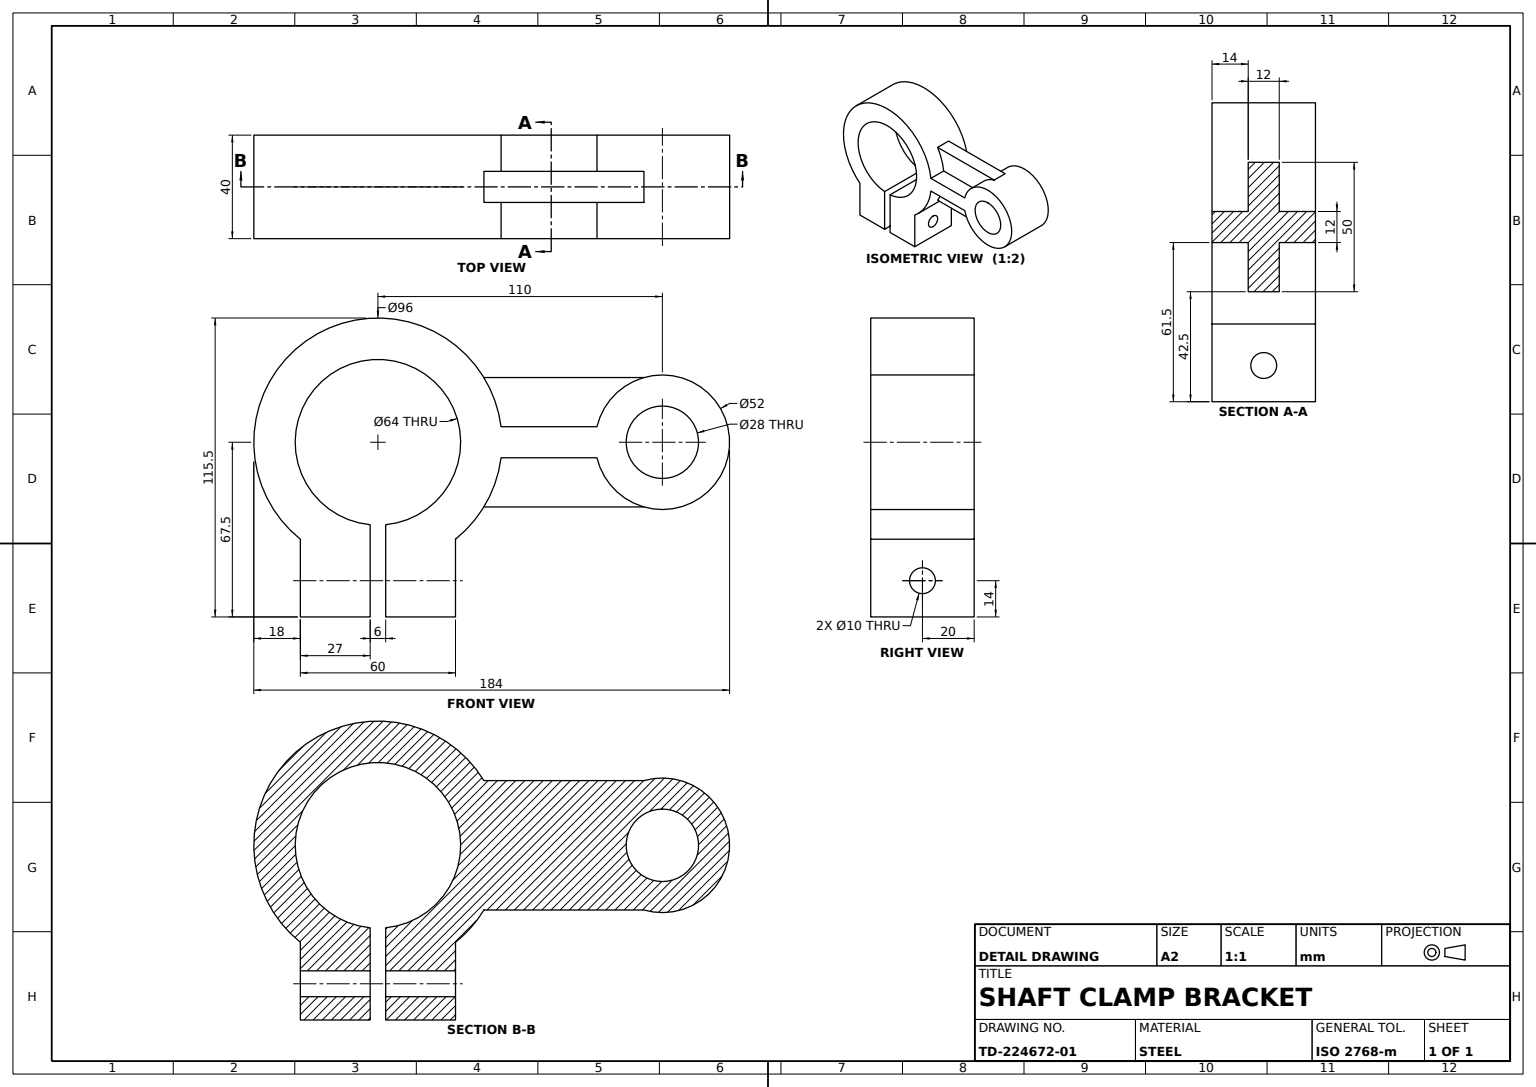
ISO-10303-21;
HEADER;
FILE_DESCRIPTION((''),'2;1');
FILE_NAME('','',(''),(''),'','','');
FILE_SCHEMA(('AUTOMOTIVE_DESIGN'));
ENDSEC;
DATA;
#1=APPLICATION_CONTEXT('');
#2=PRODUCT_CONTEXT('',#1,'mechanical');
#3=PRODUCT('','','',(#2));
#4=PRODUCT_DEFINITION_FORMATION('','',#3);
#5=PRODUCT_DEFINITION_CONTEXT('',#1,'design');
#6=PRODUCT_DEFINITION('','',#4,#5);
#7=PRODUCT_DEFINITION_SHAPE('','',#6);
#8=(LENGTH_UNIT()NAMED_UNIT(*)SI_UNIT(.MILLI.,.METRE.));
#9=(NAMED_UNIT(*)PLANE_ANGLE_UNIT()SI_UNIT($,.RADIAN.));
#10=(NAMED_UNIT(*)SI_UNIT($,.STERADIAN.)SOLID_ANGLE_UNIT());
#11=UNCERTAINTY_MEASURE_WITH_UNIT(LENGTH_MEASURE(0.005),#8,'distance_accuracy_value','');
#12=(GEOMETRIC_REPRESENTATION_CONTEXT(3)GLOBAL_UNCERTAINTY_ASSIGNED_CONTEXT((#11))GLOBAL_UNIT_ASSIGNED_CONTEXT((#8,#9,#10))REPRESENTATION_CONTEXT('',''));
#13=CARTESIAN_POINT('',(40.975602,-6.,-25.));
#14=VERTEX_POINT('',#13);
#15=CARTESIAN_POINT('',(40.975602,6.,-25.));
#16=VERTEX_POINT('',#15);
#17=CARTESIAN_POINT('',(40.975602,-20.,-25.));
#18=DIRECTION('',(0.,1.,0.));
#19=VECTOR('',#18,1000.);
#20=LINE('',#17,#19);
#21=EDGE_CURVE('',#14,#16,#20,.T.);
#22=ORIENTED_EDGE('',*,*,#21,.T.);
#23=CARTESIAN_POINT('',(102.858572,6.,-25.));
#24=VERTEX_POINT('',#23);
#25=CARTESIAN_POINT('',(35.,6.,-25.));
#26=DIRECTION('',(1.,0.,0.));
#27=VECTOR('',#26,1000.);
#28=LINE('',#25,#27);
#29=EDGE_CURVE('',#16,#24,#28,.T.);
#30=ORIENTED_EDGE('',*,*,#29,.T.);
#31=CARTESIAN_POINT('',(102.858572,-6.,-25.));
#32=VERTEX_POINT('',#31);
#33=CARTESIAN_POINT('',(102.858572,-20.,-25.));
#34=LINE('',#33,#19);
#35=EDGE_CURVE('',#32,#24,#34,.T.);
#36=ORIENTED_EDGE('',*,*,#35,.F.);
#37=CARTESIAN_POINT('',(35.,-6.,-25.));
#38=LINE('',#37,#27);
#39=EDGE_CURVE('',#14,#32,#38,.T.);
#40=ORIENTED_EDGE('',*,*,#39,.F.);
#41=EDGE_LOOP('',(#22,#30,#36,#40));
#42=FACE_BOUND('',#41,.T.);
#43=DIRECTION('',(0.,0.,1.));
#44=AXIS2_PLACEMENT_3D('',#37,#43,#26);
#45=PLANE('',#44);
#46=ADVANCED_FACE('',(#42),#45,.F.);
#47=CARTESIAN_POINT('',(30.,-20.,-37.469988));
#48=VERTEX_POINT('',#47);
#49=CARTESIAN_POINT('',(30.,20.,-37.469988));
#50=VERTEX_POINT('',#49);
#51=LINE('',#47,#19);
#52=EDGE_CURVE('',#48,#50,#51,.T.);
#53=ORIENTED_EDGE('',*,*,#52,.F.);
#54=CARTESIAN_POINT('',(30.,-20.,-67.5));
#55=VERTEX_POINT('',#54);
#56=VECTOR('',#43,1000.);
#57=LINE('',#54,#56);
#58=EDGE_CURVE('',#55,#48,#57,.T.);
#59=ORIENTED_EDGE('',*,*,#58,.F.);
#60=CARTESIAN_POINT('',(30.,20.,-67.5));
#61=VERTEX_POINT('',#60);
#62=LINE('',#54,#19);
#63=EDGE_CURVE('',#55,#61,#62,.T.);
#64=ORIENTED_EDGE('',*,*,#63,.T.);
#65=LINE('',#60,#56);
#66=EDGE_CURVE('',#61,#50,#65,.T.);
#67=ORIENTED_EDGE('',*,*,#66,.T.);
#68=EDGE_LOOP('',(#53,#59,#64,#67));
#69=FACE_BOUND('',#68,.T.);
#70=CARTESIAN_POINT('',(30.,0.,-48.5));
#71=VERTEX_POINT('',#70);
#72=CARTESIAN_POINT('',(30.,0.,-53.5));
#73=DIRECTION('',(-1.,0.,0.));
#74=AXIS2_PLACEMENT_3D('',#72,#73,#43);
#75=CIRCLE('',#74,5.);
#76=EDGE_CURVE('',#71,#71,#75,.T.);
#77=ORIENTED_EDGE('',*,*,#76,.T.);
#78=EDGE_LOOP('',(#77));
#79=FACE_BOUND('',#78,.T.);
#80=AXIS2_PLACEMENT_3D('',#54,#73,#43);
#81=PLANE('',#80);
#82=ADVANCED_FACE('',(#69,#79),#81,.F.);
#83=CARTESIAN_POINT('',(-30.,20.,-67.5));
#84=VERTEX_POINT('',#83);
#85=CARTESIAN_POINT('',(-3.,20.,-67.5));
#86=VERTEX_POINT('',#85);
#87=LINE('',#83,#27);
#88=EDGE_CURVE('',#84,#86,#87,.T.);
#89=ORIENTED_EDGE('',*,*,#88,.T.);
#90=CARTESIAN_POINT('',(-3.,-20.,-67.5));
#91=VERTEX_POINT('',#90);
#92=DIRECTION('',(0.,-1.,0.));
#93=VECTOR('',#92,1000.);
#94=LINE('',#90,#93);
#95=EDGE_CURVE('',#86,#91,#94,.T.);
#96=ORIENTED_EDGE('',*,*,#95,.T.);
#97=CARTESIAN_POINT('',(-30.,-20.,-67.5));
#98=VERTEX_POINT('',#97);
#99=LINE('',#97,#27);
#100=EDGE_CURVE('',#98,#91,#99,.T.);
#101=ORIENTED_EDGE('',*,*,#100,.F.);
#102=LINE('',#97,#19);
#103=EDGE_CURVE('',#98,#84,#102,.T.);
#104=ORIENTED_EDGE('',*,*,#103,.T.);
#105=EDGE_LOOP('',(#89,#96,#101,#104));
#106=FACE_BOUND('',#105,.T.);
#107=AXIS2_PLACEMENT_3D('',#97,#43,#26);
#108=PLANE('',#107);
#109=ADVANCED_FACE('',(#106),#108,.F.);
#110=CARTESIAN_POINT('',(-3.,0.,-48.5));
#111=VERTEX_POINT('',#110);
#112=CARTESIAN_POINT('',(-3.,0.,-53.5));
#113=AXIS2_PLACEMENT_3D('',#112,#73,#43);
#114=CIRCLE('',#113,5.);
#115=EDGE_CURVE('',#111,#111,#114,.T.);
#116=ORIENTED_EDGE('',*,*,#115,.F.);
#117=EDGE_LOOP('',(#116));
#118=FACE_BOUND('',#117,.T.);
#119=CARTESIAN_POINT('',(-30.,0.,-58.5));
#120=VERTEX_POINT('',#119);
#121=CARTESIAN_POINT('',(-30.,0.,-53.5));
#122=DIRECTION('',(0.,0.,-1.));
#123=AXIS2_PLACEMENT_3D('',#121,#26,#122);
#124=CIRCLE('',#123,5.);
#125=EDGE_CURVE('',#120,#120,#124,.T.);
#126=ORIENTED_EDGE('',*,*,#125,.F.);
#127=EDGE_LOOP('',(#126));
#128=FACE_BOUND('',#127,.T.);
#129=CYLINDRICAL_SURFACE('',#74,5.);
#130=ADVANCED_FACE('',(#118,#128),#129,.F.);
#131=CARTESIAN_POINT('',(-3.,20.,-31.859065));
#132=VERTEX_POINT('',#131);
#133=CARTESIAN_POINT('',(-3.,-20.,-31.859065));
#134=VERTEX_POINT('',#133);
#135=LINE('',#133,#19);
#136=EDGE_CURVE('',#132,#134,#135,.F.);
#137=ORIENTED_EDGE('',*,*,#136,.F.);
#138=CARTESIAN_POINT('',(3.,20.,-31.859065));
#139=VERTEX_POINT('',#138);
#140=CARTESIAN_POINT('',(0.,20.,0.));
#141=AXIS2_PLACEMENT_3D('',#140,#92,#122);
#142=CIRCLE('',#141,32.);
#143=EDGE_CURVE('',#139,#132,#142,.T.);
#144=ORIENTED_EDGE('',*,*,#143,.F.);
#145=CARTESIAN_POINT('',(3.,-20.,-31.859065));
#146=VERTEX_POINT('',#145);
#147=LINE('',#145,#19);
#148=EDGE_CURVE('',#146,#139,#147,.T.);
#149=ORIENTED_EDGE('',*,*,#148,.F.);
#150=CARTESIAN_POINT('',(0.,-20.,0.));
#151=AXIS2_PLACEMENT_3D('',#150,#18,#43);
#152=CIRCLE('',#151,32.);
#153=EDGE_CURVE('',#134,#146,#152,.T.);
#154=ORIENTED_EDGE('',*,*,#153,.F.);
#155=EDGE_LOOP('',(#137,#144,#149,#154));
#156=FACE_BOUND('',#155,.T.);
#157=CYLINDRICAL_SURFACE('',#151,32.);
#158=ADVANCED_FACE('',(#156),#157,.F.);
#159=CARTESIAN_POINT('',(84.701779,6.,-6.));
#160=VERTEX_POINT('',#159);
#161=CARTESIAN_POINT('',(47.623524,6.,-6.));
#162=VERTEX_POINT('',#161);
#163=CARTESIAN_POINT('',(0.,6.,-6.));
#164=VECTOR('',#73,1000.);
#165=LINE('',#163,#164);
#166=EDGE_CURVE('',#160,#162,#165,.T.);
#167=ORIENTED_EDGE('',*,*,#166,.T.);
#168=CARTESIAN_POINT('',(47.623524,20.,-6.));
#169=VERTEX_POINT('',#168);
#170=CARTESIAN_POINT('',(47.623524,-20.,-6.));
#171=LINE('',#170,#19);
#172=EDGE_CURVE('',#162,#169,#171,.T.);
#173=ORIENTED_EDGE('',*,*,#172,.T.);
#174=CARTESIAN_POINT('',(84.701779,20.,-6.));
#175=VERTEX_POINT('',#174);
#176=CARTESIAN_POINT('',(90.,20.,-6.));
#177=LINE('',#176,#164);
#178=EDGE_CURVE('',#175,#169,#177,.T.);
#179=ORIENTED_EDGE('',*,*,#178,.F.);
#180=CARTESIAN_POINT('',(84.701779,-20.,-6.));
#181=LINE('',#180,#19);
#182=EDGE_CURVE('',#175,#160,#181,.F.);
#183=ORIENTED_EDGE('',*,*,#182,.T.);
#184=EDGE_LOOP('',(#167,#173,#179,#183));
#185=FACE_BOUND('',#184,.T.);
#186=CARTESIAN_POINT('',(0.,0.,-6.));
#187=AXIS2_PLACEMENT_3D('',#186,#43,#26);
#188=PLANE('',#187);
#189=ADVANCED_FACE('',(#185),#188,.F.);
#190=CARTESIAN_POINT('',(40.975602,6.,25.));
#191=VERTEX_POINT('',#190);
#192=CARTESIAN_POINT('',(40.975602,-6.,25.));
#193=VERTEX_POINT('',#192);
#194=CARTESIAN_POINT('',(40.975602,-20.,25.));
#195=LINE('',#194,#19);
#196=EDGE_CURVE('',#191,#193,#195,.F.);
#197=ORIENTED_EDGE('',*,*,#196,.T.);
#198=CARTESIAN_POINT('',(102.858572,-6.,25.));
#199=VERTEX_POINT('',#198);
#200=CARTESIAN_POINT('',(110.,-6.,25.));
#201=LINE('',#200,#164);
#202=EDGE_CURVE('',#199,#193,#201,.T.);
#203=ORIENTED_EDGE('',*,*,#202,.F.);
#204=CARTESIAN_POINT('',(102.858572,6.,25.));
#205=VERTEX_POINT('',#204);
#206=CARTESIAN_POINT('',(102.858572,-20.,25.));
#207=LINE('',#206,#19);
#208=EDGE_CURVE('',#205,#199,#207,.F.);
#209=ORIENTED_EDGE('',*,*,#208,.F.);
#210=CARTESIAN_POINT('',(110.,6.,25.));
#211=LINE('',#210,#164);
#212=EDGE_CURVE('',#205,#191,#211,.T.);
#213=ORIENTED_EDGE('',*,*,#212,.T.);
#214=EDGE_LOOP('',(#197,#203,#209,#213));
#215=FACE_BOUND('',#214,.T.);
#216=AXIS2_PLACEMENT_3D('',#200,#122,#73);
#217=PLANE('',#216);
#218=ADVANCED_FACE('',(#215),#217,.F.);
#219=CARTESIAN_POINT('',(110.,-20.,14.));
#220=VERTEX_POINT('',#219);
#221=CARTESIAN_POINT('',(110.,-20.,0.));
#222=AXIS2_PLACEMENT_3D('',#221,#18,#43);
#223=CIRCLE('',#222,14.);
#224=EDGE_CURVE('',#220,#220,#223,.T.);
#225=ORIENTED_EDGE('',*,*,#224,.F.);
#226=EDGE_LOOP('',(#225));
#227=FACE_BOUND('',#226,.T.);
#228=CARTESIAN_POINT('',(110.,20.,-14.));
#229=VERTEX_POINT('',#228);
#230=CARTESIAN_POINT('',(110.,20.,0.));
#231=AXIS2_PLACEMENT_3D('',#230,#92,#122);
#232=CIRCLE('',#231,14.);
#233=EDGE_CURVE('',#229,#229,#232,.T.);
#234=ORIENTED_EDGE('',*,*,#233,.F.);
#235=EDGE_LOOP('',(#234));
#236=FACE_BOUND('',#235,.T.);
#237=CYLINDRICAL_SURFACE('',#222,14.);
#238=ADVANCED_FACE('',(#227,#236),#237,.F.);
#239=CARTESIAN_POINT('',(3.,-20.,-67.5));
#240=VERTEX_POINT('',#239);
#241=CARTESIAN_POINT('',(3.,20.,-67.5));
#242=VERTEX_POINT('',#241);
#243=LINE('',#239,#19);
#244=EDGE_CURVE('',#240,#242,#243,.T.);
#245=ORIENTED_EDGE('',*,*,#244,.F.);
#246=CARTESIAN_POINT('',(3.,-20.,0.));
#247=LINE('',#246,#56);
#248=EDGE_CURVE('',#240,#146,#247,.T.);
#249=ORIENTED_EDGE('',*,*,#248,.T.);
#250=ORIENTED_EDGE('',*,*,#148,.T.);
#251=CARTESIAN_POINT('',(3.,20.,0.));
#252=LINE('',#251,#56);
#253=EDGE_CURVE('',#242,#139,#252,.T.);
#254=ORIENTED_EDGE('',*,*,#253,.F.);
#255=EDGE_LOOP('',(#245,#249,#250,#254));
#256=FACE_BOUND('',#255,.T.);
#257=CARTESIAN_POINT('',(3.,0.,-58.5));
#258=VERTEX_POINT('',#257);
#259=CARTESIAN_POINT('',(3.,0.,-53.5));
#260=AXIS2_PLACEMENT_3D('',#259,#26,#122);
#261=CIRCLE('',#260,5.);
#262=EDGE_CURVE('',#258,#258,#261,.T.);
#263=ORIENTED_EDGE('',*,*,#262,.T.);
#264=EDGE_LOOP('',(#263));
#265=FACE_BOUND('',#264,.T.);
#266=CARTESIAN_POINT('',(3.,-25.,-30.384328));
#267=AXIS2_PLACEMENT_3D('',#266,#26,#122);
#268=PLANE('',#267);
#269=ADVANCED_FACE('',(#256,#265),#268,.F.);
#270=ORIENTED_EDGE('',*,*,#208,.T.);
#271=CARTESIAN_POINT('',(84.701779,-6.,6.));
#272=VERTEX_POINT('',#271);
#273=CARTESIAN_POINT('',(110.,-6.,0.));
#274=AXIS2_PLACEMENT_3D('',#273,#92,#122);
#275=CIRCLE('',#274,26.);
#276=EDGE_CURVE('',#272,#199,#275,.F.);
#277=ORIENTED_EDGE('',*,*,#276,.F.);
#278=CARTESIAN_POINT('',(84.701779,-20.,6.));
#279=VERTEX_POINT('',#278);
#280=LINE('',#278,#19);
#281=EDGE_CURVE('',#272,#279,#280,.F.);
#282=ORIENTED_EDGE('',*,*,#281,.T.);
#283=VERTEX_POINT('',#180);
#284=AXIS2_PLACEMENT_3D('',#221,#92,#26);
#285=CIRCLE('',#284,26.);
#286=EDGE_CURVE('',#283,#279,#285,.T.);
#287=ORIENTED_EDGE('',*,*,#286,.F.);
#288=CARTESIAN_POINT('',(84.701779,-6.,-6.));
#289=VERTEX_POINT('',#288);
#290=EDGE_CURVE('',#289,#283,#181,.F.);
#291=ORIENTED_EDGE('',*,*,#290,.F.);
#292=EDGE_CURVE('',#32,#289,#275,.F.);
#293=ORIENTED_EDGE('',*,*,#292,.F.);
#294=ORIENTED_EDGE('',*,*,#35,.T.);
#295=CARTESIAN_POINT('',(110.,6.,0.));
#296=AXIS2_PLACEMENT_3D('',#295,#92,#122);
#297=CIRCLE('',#296,26.);
#298=EDGE_CURVE('',#24,#160,#297,.F.);
#299=ORIENTED_EDGE('',*,*,#298,.T.);
#300=ORIENTED_EDGE('',*,*,#182,.F.);
#301=CARTESIAN_POINT('',(84.701779,20.,6.));
#302=VERTEX_POINT('',#301);
#303=AXIS2_PLACEMENT_3D('',#230,#92,#26);
#304=CIRCLE('',#303,26.);
#305=EDGE_CURVE('',#175,#302,#304,.T.);
#306=ORIENTED_EDGE('',*,*,#305,.T.);
#307=CARTESIAN_POINT('',(84.701779,6.,6.));
#308=VERTEX_POINT('',#307);
#309=EDGE_CURVE('',#302,#308,#280,.F.);
#310=ORIENTED_EDGE('',*,*,#309,.T.);
#311=EDGE_CURVE('',#308,#205,#297,.F.);
#312=ORIENTED_EDGE('',*,*,#311,.T.);
#313=EDGE_LOOP('',(#270,#277,#282,#287,#291,#293,#294,#299,#300,#306,#310,#312));
#314=FACE_BOUND('',#313,.T.);
#315=CYLINDRICAL_SURFACE('',#222,26.);
#316=ADVANCED_FACE('',(#314),#315,.T.);
#317=CARTESIAN_POINT('',(47.623524,-6.,-6.));
#318=VERTEX_POINT('',#317);
#319=CARTESIAN_POINT('',(0.,-6.,-6.));
#320=LINE('',#319,#164);
#321=EDGE_CURVE('',#289,#318,#320,.T.);
#322=ORIENTED_EDGE('',*,*,#321,.F.);
#323=ORIENTED_EDGE('',*,*,#290,.T.);
#324=VERTEX_POINT('',#170);
#325=CARTESIAN_POINT('',(40.,-20.,-6.));
#326=LINE('',#325,#27);
#327=EDGE_CURVE('',#324,#283,#326,.T.);
#328=ORIENTED_EDGE('',*,*,#327,.F.);
#329=EDGE_CURVE('',#324,#318,#171,.T.);
#330=ORIENTED_EDGE('',*,*,#329,.T.);
#331=EDGE_LOOP('',(#322,#323,#328,#330));
#332=FACE_BOUND('',#331,.T.);
#333=ADVANCED_FACE('',(#332),#188,.F.);
#334=ORIENTED_EDGE('',*,*,#63,.F.);
#335=EDGE_CURVE('',#240,#55,#99,.T.);
#336=ORIENTED_EDGE('',*,*,#335,.F.);
#337=ORIENTED_EDGE('',*,*,#244,.T.);
#338=EDGE_CURVE('',#242,#61,#87,.T.);
#339=ORIENTED_EDGE('',*,*,#338,.T.);
#340=EDGE_LOOP('',(#334,#336,#337,#339));
#341=FACE_BOUND('',#340,.T.);
#342=ADVANCED_FACE('',(#341),#108,.F.);
#343=CARTESIAN_POINT('',(-30.,-20.,-37.469988));
#344=VERTEX_POINT('',#343);
#345=VECTOR('',#122,1000.);
#346=LINE('',#343,#345);
#347=EDGE_CURVE('',#344,#98,#346,.T.);
#348=ORIENTED_EDGE('',*,*,#347,.F.);
#349=CARTESIAN_POINT('',(-30.,20.,-37.469988));
#350=VERTEX_POINT('',#349);
#351=LINE('',#343,#19);
#352=EDGE_CURVE('',#344,#350,#351,.T.);
#353=ORIENTED_EDGE('',*,*,#352,.T.);
#354=LINE('',#349,#345);
#355=EDGE_CURVE('',#350,#84,#354,.T.);
#356=ORIENTED_EDGE('',*,*,#355,.T.);
#357=ORIENTED_EDGE('',*,*,#103,.F.);
#358=EDGE_LOOP('',(#348,#353,#356,#357));
#359=FACE_BOUND('',#358,.T.);
#360=ORIENTED_EDGE('',*,*,#125,.T.);
#361=EDGE_LOOP('',(#360));
#362=FACE_BOUND('',#361,.T.);
#363=AXIS2_PLACEMENT_3D('',#343,#26,#122);
#364=PLANE('',#363);
#365=ADVANCED_FACE('',(#359,#362),#364,.F.);
#366=ORIENTED_EDGE('',*,*,#298,.F.);
#367=ORIENTED_EDGE('',*,*,#29,.F.);
#368=CARTESIAN_POINT('',(0.,6.,0.));
#369=AXIS2_PLACEMENT_3D('',#368,#92,#122);
#370=CIRCLE('',#369,48.);
#371=EDGE_CURVE('',#16,#162,#370,.T.);
#372=ORIENTED_EDGE('',*,*,#371,.T.);
#373=ORIENTED_EDGE('',*,*,#166,.F.);
#374=EDGE_LOOP('',(#366,#367,#372,#373));
#375=FACE_BOUND('',#374,.T.);
#376=PLANE('',#369);
#377=ADVANCED_FACE('',(#375),#376,.F.);
#378=ORIENTED_EDGE('',*,*,#233,.T.);
#379=EDGE_LOOP('',(#378));
#380=FACE_BOUND('',#379,.T.);
#381=CARTESIAN_POINT('',(47.623524,20.,6.));
#382=VERTEX_POINT('',#381);
#383=AXIS2_PLACEMENT_3D('',#140,#92,#26);
#384=CIRCLE('',#383,48.);
#385=EDGE_CURVE('',#382,#350,#384,.T.);
#386=ORIENTED_EDGE('',*,*,#385,.F.);
#387=CARTESIAN_POINT('',(90.,20.,6.));
#388=LINE('',#387,#164);
#389=EDGE_CURVE('',#302,#382,#388,.T.);
#390=ORIENTED_EDGE('',*,*,#389,.F.);
#391=ORIENTED_EDGE('',*,*,#305,.F.);
#392=ORIENTED_EDGE('',*,*,#178,.T.);
#393=EDGE_CURVE('',#50,#169,#384,.T.);
#394=ORIENTED_EDGE('',*,*,#393,.F.);
#395=ORIENTED_EDGE('',*,*,#66,.F.);
#396=ORIENTED_EDGE('',*,*,#338,.F.);
#397=ORIENTED_EDGE('',*,*,#253,.T.);
#398=ORIENTED_EDGE('',*,*,#143,.T.);
#399=CARTESIAN_POINT('',(-3.,20.,0.));
#400=LINE('',#399,#345);
#401=EDGE_CURVE('',#132,#86,#400,.T.);
#402=ORIENTED_EDGE('',*,*,#401,.T.);
#403=ORIENTED_EDGE('',*,*,#88,.F.);
#404=ORIENTED_EDGE('',*,*,#355,.F.);
#405=EDGE_LOOP('',(#386,#390,#391,#392,#394,#395,#396,#397,#398,#402,#403,#404));
#406=FACE_BOUND('',#405,.T.);
#407=PLANE('',#141);
#408=ADVANCED_FACE('',(#380,#406),#407,.F.);
#409=CARTESIAN_POINT('',(47.623524,-6.,6.));
#410=VERTEX_POINT('',#409);
#411=CARTESIAN_POINT('',(0.,-6.,0.));
#412=AXIS2_PLACEMENT_3D('',#411,#92,#122);
#413=CIRCLE('',#412,48.);
#414=EDGE_CURVE('',#410,#193,#413,.T.);
#415=ORIENTED_EDGE('',*,*,#414,.F.);
#416=CARTESIAN_POINT('',(0.,-6.,6.));
#417=LINE('',#416,#164);
#418=EDGE_CURVE('',#272,#410,#417,.T.);
#419=ORIENTED_EDGE('',*,*,#418,.F.);
#420=ORIENTED_EDGE('',*,*,#276,.T.);
#421=ORIENTED_EDGE('',*,*,#202,.T.);
#422=EDGE_LOOP('',(#415,#419,#420,#421));
#423=FACE_BOUND('',#422,.T.);
#424=PLANE('',#412);
#425=ADVANCED_FACE('',(#423),#424,.T.);
#426=CARTESIAN_POINT('',(47.623524,-20.,6.));
#427=VERTEX_POINT('',#426);
#428=LINE('',#426,#19);
#429=EDGE_CURVE('',#427,#410,#428,.T.);
#430=ORIENTED_EDGE('',*,*,#429,.F.);
#431=CARTESIAN_POINT('',(40.,-20.,6.));
#432=LINE('',#431,#27);
#433=EDGE_CURVE('',#427,#279,#432,.T.);
#434=ORIENTED_EDGE('',*,*,#433,.T.);
#435=ORIENTED_EDGE('',*,*,#281,.F.);
#436=ORIENTED_EDGE('',*,*,#418,.T.);
#437=EDGE_LOOP('',(#430,#434,#435,#436));
#438=FACE_BOUND('',#437,.T.);
#439=CARTESIAN_POINT('',(0.,0.,6.));
#440=AXIS2_PLACEMENT_3D('',#439,#43,#26);
#441=PLANE('',#440);
#442=ADVANCED_FACE('',(#438),#441,.T.);
#443=CARTESIAN_POINT('',(47.623524,6.,6.));
#444=VERTEX_POINT('',#443);
#445=CARTESIAN_POINT('',(0.,6.,6.));
#446=LINE('',#445,#164);
#447=EDGE_CURVE('',#308,#444,#446,.T.);
#448=ORIENTED_EDGE('',*,*,#447,.T.);
#449=EDGE_CURVE('',#444,#191,#370,.T.);
#450=ORIENTED_EDGE('',*,*,#449,.T.);
#451=ORIENTED_EDGE('',*,*,#212,.F.);
#452=ORIENTED_EDGE('',*,*,#311,.F.);
#453=EDGE_LOOP('',(#448,#450,#451,#452));
#454=FACE_BOUND('',#453,.T.);
#455=ADVANCED_FACE('',(#454),#376,.F.);
#456=AXIS2_PLACEMENT_3D('',#150,#92,#26);
#457=CIRCLE('',#456,48.);
#458=EDGE_CURVE('',#427,#344,#457,.T.);
#459=ORIENTED_EDGE('',*,*,#458,.F.);
#460=ORIENTED_EDGE('',*,*,#429,.T.);
#461=ORIENTED_EDGE('',*,*,#414,.T.);
#462=ORIENTED_EDGE('',*,*,#196,.F.);
#463=ORIENTED_EDGE('',*,*,#449,.F.);
#464=EDGE_CURVE('',#444,#382,#428,.T.);
#465=ORIENTED_EDGE('',*,*,#464,.T.);
#466=ORIENTED_EDGE('',*,*,#385,.T.);
#467=ORIENTED_EDGE('',*,*,#352,.F.);
#468=EDGE_LOOP('',(#459,#460,#461,#462,#463,#465,#466,#467));
#469=FACE_BOUND('',#468,.T.);
#470=CYLINDRICAL_SURFACE('',#151,48.);
#471=ADVANCED_FACE('',(#469),#470,.T.);
#472=CARTESIAN_POINT('',(-3.,-20.,0.));
#473=LINE('',#472,#345);
#474=EDGE_CURVE('',#134,#91,#473,.T.);
#475=ORIENTED_EDGE('',*,*,#474,.T.);
#476=ORIENTED_EDGE('',*,*,#95,.F.);
#477=ORIENTED_EDGE('',*,*,#401,.F.);
#478=ORIENTED_EDGE('',*,*,#136,.T.);
#479=EDGE_LOOP('',(#475,#476,#477,#478));
#480=FACE_BOUND('',#479,.T.);
#481=ORIENTED_EDGE('',*,*,#115,.T.);
#482=EDGE_LOOP('',(#481));
#483=FACE_BOUND('',#482,.T.);
#484=CARTESIAN_POINT('',(-3.,-25.,-75.251731));
#485=AXIS2_PLACEMENT_3D('',#484,#73,#43);
#486=PLANE('',#485);
#487=ADVANCED_FACE('',(#480,#483),#486,.F.);
#488=ORIENTED_EDGE('',*,*,#39,.T.);
#489=ORIENTED_EDGE('',*,*,#292,.T.);
#490=ORIENTED_EDGE('',*,*,#321,.T.);
#491=EDGE_CURVE('',#14,#318,#413,.T.);
#492=ORIENTED_EDGE('',*,*,#491,.F.);
#493=EDGE_LOOP('',(#488,#489,#490,#492));
#494=FACE_BOUND('',#493,.T.);
#495=ADVANCED_FACE('',(#494),#424,.T.);
#496=ORIENTED_EDGE('',*,*,#21,.F.);
#497=ORIENTED_EDGE('',*,*,#491,.T.);
#498=ORIENTED_EDGE('',*,*,#329,.F.);
#499=EDGE_CURVE('',#48,#324,#457,.T.);
#500=ORIENTED_EDGE('',*,*,#499,.F.);
#501=ORIENTED_EDGE('',*,*,#52,.T.);
#502=ORIENTED_EDGE('',*,*,#393,.T.);
#503=ORIENTED_EDGE('',*,*,#172,.F.);
#504=ORIENTED_EDGE('',*,*,#371,.F.);
#505=EDGE_LOOP('',(#496,#497,#498,#500,#501,#502,#503,#504));
#506=FACE_BOUND('',#505,.T.);
#507=ADVANCED_FACE('',(#506),#470,.T.);
#508=ORIENTED_EDGE('',*,*,#447,.F.);
#509=ORIENTED_EDGE('',*,*,#309,.F.);
#510=ORIENTED_EDGE('',*,*,#389,.T.);
#511=ORIENTED_EDGE('',*,*,#464,.F.);
#512=EDGE_LOOP('',(#508,#509,#510,#511));
#513=FACE_BOUND('',#512,.T.);
#514=ADVANCED_FACE('',(#513),#441,.T.);
#515=ORIENTED_EDGE('',*,*,#76,.F.);
#516=EDGE_LOOP('',(#515));
#517=FACE_BOUND('',#516,.T.);
#518=ORIENTED_EDGE('',*,*,#262,.F.);
#519=EDGE_LOOP('',(#518));
#520=FACE_BOUND('',#519,.T.);
#521=ADVANCED_FACE('',(#517,#520),#129,.F.);
#522=ORIENTED_EDGE('',*,*,#224,.T.);
#523=EDGE_LOOP('',(#522));
#524=FACE_BOUND('',#523,.T.);
#525=ORIENTED_EDGE('',*,*,#327,.T.);
#526=ORIENTED_EDGE('',*,*,#286,.T.);
#527=ORIENTED_EDGE('',*,*,#433,.F.);
#528=ORIENTED_EDGE('',*,*,#458,.T.);
#529=ORIENTED_EDGE('',*,*,#347,.T.);
#530=ORIENTED_EDGE('',*,*,#100,.T.);
#531=ORIENTED_EDGE('',*,*,#474,.F.);
#532=ORIENTED_EDGE('',*,*,#153,.T.);
#533=ORIENTED_EDGE('',*,*,#248,.F.);
#534=ORIENTED_EDGE('',*,*,#335,.T.);
#535=ORIENTED_EDGE('',*,*,#58,.T.);
#536=ORIENTED_EDGE('',*,*,#499,.T.);
#537=EDGE_LOOP('',(#525,#526,#527,#528,#529,#530,#531,#532,#533,#534,#535,#536));
#538=FACE_BOUND('',#537,.T.);
#539=AXIS2_PLACEMENT_3D('',#150,#92,#122);
#540=PLANE('',#539);
#541=ADVANCED_FACE('',(#524,#538),#540,.T.);
#542=CLOSED_SHELL('',(#46,#82,#109,#130,#158,#189,#218,#238,#269,#316,#333,#342,#365,#377,#408,#425,#442,#455,#471,#487,#495,#507,#514,#521,#541));
#543=MANIFOLD_SOLID_BREP('',#542);
#544=ADVANCED_BREP_SHAPE_REPRESENTATION('',(#543),#12);
#545=SHAPE_DEFINITION_REPRESENTATION(#7,#544);
ENDSEC;
END-ISO-10303-21;
